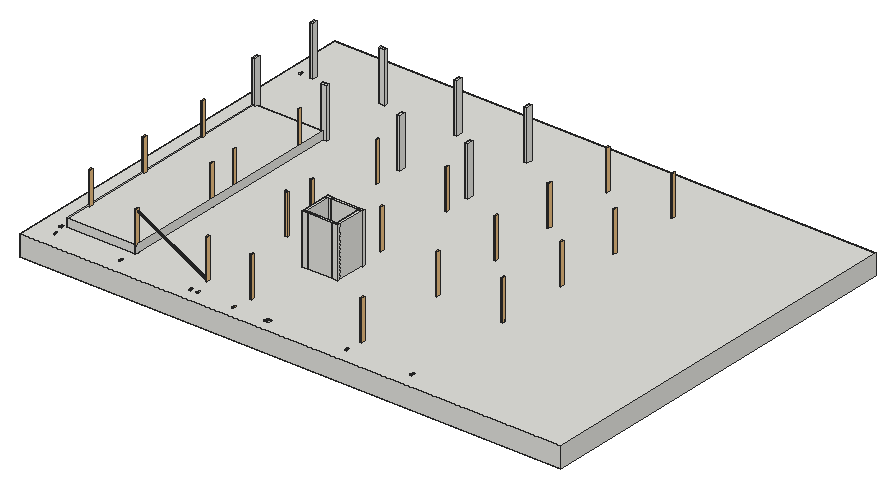
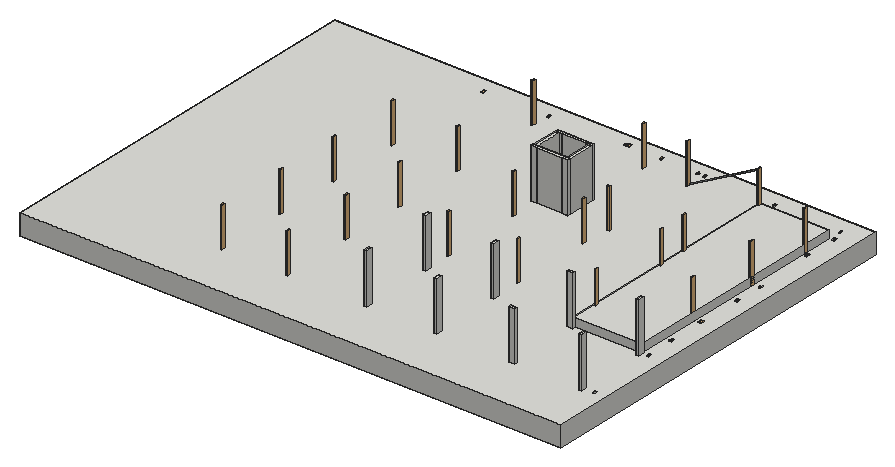
# SketchUp Ruby script. Lengths in millimetres.
U = 1.mm
M = Sketchup.active_model
def pt(a) = Geom::Point3d.new(a.map { |v| v * U })
def face(e, loops, mat)
  f = e.add_face(loops[0].map { |a| pt(a) })
  loops[1..].each { |l| e.add_face(l.map { |a| pt(a) }).erase! }
  f.material = f.back_material = mat if mat
  f
end
# faces: each face lists its corners as indices into pts; further lists are holes
def faces(e, pts, list, mat = nil) = list.each { |f| face(e, (f[0].is_a?(Array) ? f : [f]).map { |l| l.map { |i| pts[i] } }, mat) }
# xy, xz, yz: faces in a plane at the given z, y or x. An outline is a flat list of corners, or four numbers for a rectangle; further outlines are holes
def ring(l) = l.size == 4 ? [[l[0], l[1]], [l[2], l[1]], [l[2], l[3]], [l[0], l[3]]] : l.each_slice(2).to_a
def flat(e, list, mat, &to3) = list.each { |f| face(e, (f[0].is_a?(Array) ? f : [f]).map { |l| ring(l).map { |u, v| to3.(u, v) } }, mat) }
def xy(e, z, list, mat = nil) = flat(e, list, mat) { |x, y| [x, y, z] }
def xz(e, y, list, mat = nil) = flat(e, list, mat) { |x, z| [x, y, z] }
def yz(e, x, list, mat = nil) = flat(e, list, mat) { |y, z| [x, y, z] }
def lines(e, pts, list) = list.each { |a, b| e.add_line(pt(pts[a]), pt(pts[b])) }
# prism: a flat outline (further loops are holes) pulled along v
def prism(e, loops, v, mat = nil)
  f = face(e, loops, mat); d = Geom::Vector3d.new(v.map { |x| x * U })
  f.pushpull(f.normal.samedirection?(d) ? d.length : -d.length)
end
def box(e, o, s, mat = nil) = prism(e, [[o, [o[0] + s[0], o[1], o[2]], [o[0] + s[0], o[1] + s[1], o[2]], [o[0], o[1] + s[1], o[2]]]], [0, 0, s[2]], mat)
def at(x, y, z, deg = 0) = Geom::Transformation.translation(pt([x, y, z])) * Geom::Transformation.rotation(ORIGIN, Z_AXIS, deg.degrees)
def axes(o, x, y, z) = Geom::Transformation.new([*x, 0, *y, 0, *z, 0, *pt(o).to_a, 1])
def part(name) = M.definitions.add(name)
# library, detail: a bought-in or finely detailed component or shape, given as its bounding box
def library(name, o, s) = part(name).tap { |d| box(d.entities, o, s) }
def detail(e, o, s) = box(e.add_group.entities, o, s)
def put(e, d, t, mat = nil) = e.add_instance(d, t).tap { |i| i.material = mat if mat }
def group(e, t, mat = nil) = e.add_group.tap { |g| g.transformation = t; g.material = mat if mat }.entities
root = M.entities
M.materials.add("[Metal Rough]").color = [153, 157, 160]
c1 = library("8",[12,0,0],[157.3,252.5,25])
c2 = library("Group\#5",[0,0,0],[100,200,3000])
c3 = library("Group\#1",[0,0,0],[125,250,3000])
c4 = part("Group\#59")
box(c4.entities,[0,0,0],[2000,230,3746.4])
c5 = part("B ")
prism(c5.entities,[[[-1.6,0,0],[79.8,241.5,0],[119.4,241.5,0],[200.8,0,0],[166.9,0,0],[145,67.5,0],[52.7,67.5,0],[30.8,0,0]],[[136.1,94.9,0],[98.8,208.7,0],[61.6,94.9,0]]],[0,0,25])
c6 = part("B")
detail(c6.entities,[24.5,0,0],[163.8,241.5,25])
c7 = part("C")
detail(c7.entities,[10.7,0,0],[183.3,250.3,25])
c8 = part("D")
detail(c8.entities,[24.5,0,0],[190.4,241.5,25])
c9 = part("E")
prism(c9.entities,[[[24.5,0,0],[24.5,241.5,0],[175.5,241.5,0],[175.5,213,0],[56.6,213,0],[56.6,146.8,0],[167.4,146.8,0],[167.4,118.2,0],[56.6,118.2,0],[56.6,28.5,0],[175.5,28.5,0],[175.5,0,0]]],[0,0,25])
c10 = part("F")
prism(c10.entities,[[[169,213,0],[56.6,213,0],[56.6,144.8,0],[164.3,144.8,0],[164.3,116.3,0],[56.6,116.3,0],[56.6,0,0],[24.5,0,0],[24.5,241.5,0],[169,241.5,0]]],[0,0,25])
c11 = part("G")
detail(c11.entities,[10.7,0,0],[195.1,250.6,25])
c12 = part("H")
prism(c12.entities,[[[199.8,0,0],[167.7,0,0],[167.7,118.2,0],[56.6,118.2,0],[56.6,0,0],[24.5,0,0],[24.5,241.5,0],[56.6,241.5,0],[56.6,146.8,0],[167.7,146.8,0],[167.7,241.5,0],[199.8,241.5,0]]],[0,0,25])
c13 = part("1")
prism(c13.entities,[[[154.4,0,0],[36.7,0,0],[36.7,24.7,0],[80.4,24.7,0],[80.4,186.5,0],[36.7,186.5,0],[36.7,208.6,0],[58.2,210.3,0],[73.2,215.6,0],[78.5,220,0],[82.4,225.8,0],[86.5,242.3,0],[111.6,242.3,0],[111.6,24.7,0],[154.4,24.7,0]]],[0,0,25])
c14 = part("2")
prism(c14.entities,[[[166.7,0,0],[17.7,0,0],[17.7,33.9,0],[48,63.1,0],[75.9,92.1,0],[99.1,119.4,0],[113.5,140.7,0],[121.1,159.3,0],[123.6,178.4,0],[120.4,196.1,0],[111.8,208.7,0],[98.6,216,0],[82.2,218.5,0],[64.8,216.3,0],[47.8,210.9,0],[34.7,204.2,0],[24.5,197.6,0],[22.7,197.6,0],[22.7,231.9,0],[50.7,241.8,0],[68.1,245.3,0],[84.7,246.5,0],[100.6,245.4,0],[114.8,242.1,0],[127.1,236.5,0],[137.5,228.6,0],[145.9,218.9,0],[151.9,207.5,0],[155.5,194.6,0],[156.7,180,0],[153.4,153.9,0],[144.2,131.7,0],[129.8,110.8,0],[111.9,90.3,0],[77.9,56,0],[48,27.7,0],[166.7,27.7,0]]],[0,0,25])
c15 = part("4")
prism(c15.entities,[[[173.1,83,0],[144.4,83,0],[144.4,0,0],[113.2,0,0],[113.2,83,0],[6.5,83,0],[6.5,117.1,0],[114.5,241.5,0],[144.4,241.5,0],[144.4,109,0],[173.1,109,0]],[[113.2,109,0],[113.2,203.4,0],[31.8,109,0]]],[0,0,25])
c16 = part("5")
detail(c16.entities,[20.1,0,0],[143.9,246.5,25])
c17 = part("6")
detail(c17.entities,[13.8,0,0],[156.7,251.1,25])
c18 = part("7")
prism(c18.entities,[[[169.3,205.3,0],[64.9,0,0],[30.3,0,0],[140.9,213.1,0],[16.1,213.1,0],[16.1,241.5,0],[169.3,241.5,0]]],[0,0,25])
c19 = part("9")
detail(c19.entities,[10.9,0,0],[156.6,251.1,25])
c20 = library("Group\#73",[0,0,0],[16.3,16.3,61.7])
c21 = part("3")
detail(c21.entities,[15.7,0,0],[146.8,251.6,25])
g1 = group(root,at(0,2478,-1551))
box(g1,[0,-2478,0],[40875.4,29685.8,1551])
g2 = group(root,at(6833.7,2438,3000),"[Metal Rough]")
prism(g2,[[[-38.3,0,-70.3],[-38.3,80,-70.3],[5356.3,80,-3007.8],[5356.3,0,-3007.8]]],[38.3,0,70.3])
g3 = group(root,at(15878.1,7293,0))
box(g3,[0,0,0],[1833.8,230,3746.4])
g4 = group(root,at(1645,2353,0))
put(g4,c1,at(22015.6,-1306.6,0))
put(g4,c2,at(5100,9275,0))
g5 = group(g4,at(10915,17519.8,0))
box(g5,[0,0,0],[230,452.4,3740.9])
g6 = group(g4,at(5523.1,23134,0))
box(g6,[-452.4,0,0],[452.4,230,3740.9])
g7 = group(g4,at(10915,22910.9,0))
box(g7,[0,0,0],[230,452.4,3740.9])
put(g4,c3,at(5122.5,7084.8,0))
put(g4,c3,at(5122.5,0,0))
put(g4,c2,at(5100,15431,0))
g8 = group(g4,at(0,17519.8,0))
box(g8,[0,0,0],[230,452.4,3740.9])
put(g4,c3,at(13832.5,0,0))
g9 = group(g4,at(14233.1,7170,0,90))
box(g9,[0,0,0],[230,452.4,3746.4])
put(g4,c3,at(52.5,2000,0))
put(g4,c3,at(52.5,7084.8,0))
put(g4,c2,at(10980,9275,0))
put(g4,c3,at(10482.5,0,0))
put(g4,c3,at(52.5,12608,0))
g10 = group(g4,at(0,22910.9,0))
box(g10,[0,0,0],[230,452.4,3740.9])
put(g4,c3,at(10680,7347.5,0,-90))
put(g4,c2,at(10980,15431,0))
g11 = group(g4,at(5523.1,17631,0))
box(g11,[-452.4,0,0],[452.4,230,3740.9])
g12 = group(g4,at(14233.1,4940,0,90))
box(g12,[0,0,0],[230,452.4,3746.4])
g13 = group(g4,at(16175,22910.9,0))
box(g13,[0,0,0],[230,452.4,3740.9])
g14 = group(g4,at(16175,17407.9,0))
box(g14,[0,0,0],[230,452.4,3740.9])
put(g4,c2,at(16240,9275,0))
put(g4,c2,at(16240,15431,0))
g15 = group(g4,at(16519.3,4940,0,90))
box(g15,[0,0,0],[230,452.4,3746.4])
g16 = group(g4,at(16631.2,7170,0,90))
box(g16,[0,0,0],[230,452.4,3746.4])
put(g4,c3,at(22177.5,0,0))
put(g4,c3,at(22177.5,7084.8,0))
put(g4,c3,at(22177.5,12608,0))
put(g4,c3,at(22177.5,17621,0))
put(g4,c3,at(22177.5,23124,0))
put(g4,c3,at(27132.5,7084.8,0))
put(g4,c3,at(27132.5,23124,0))
put(g4,c3,at(27132.5,17621,0))
put(g4,c3,at(27132.5,12608,0))
put(root,c4,at(17934.3,9523,0,-90))
g17 = group(root,at(15878.1,9523,0))
box(g17,[0,0,0],[1945.7,230,3746.4])
put(root,c4,at(15425.7,9523,0,-90))
put(root,c5,at(813.2,25280,0))
put(root,c6,at(1082.5,19820.8,0))
put(root,c7,at(1164.7,17555.6,0))
put(root,c8,at(1211.8,14730.4,0))
put(root,c9,at(1135.2,11413.9,0))
put(root,c10,at(1081.9,9260.4,0))
put(root,c11,at(1336.6,4568.6,0))
put(root,c12,at(1257.6,2110.8,0))
put(root,c13,at(1535.1,1197.5,0))
put(root,c14,at(6569.6,1128.8,0))
put(root,c15,at(12492.4,914.9,0))
put(root,c16,at(15273.8,852.5,0))
put(root,c17,at(17748.3,824.2,0))
put(root,c18,at(17982,812.7,0))
put(root,c19,at(28541.2,1120.7,0))
g18 = group(root,at(1760,2353,0))
box(g18,[-62.5,0,0],[5195.4,17631,600])
put(root,c20,axes([28923.4,9599.9,0],[1.6,0,0],[0,1.6,0],[0,0,1.6]))
put(root,c21,at(11974.8,942.1,0))
